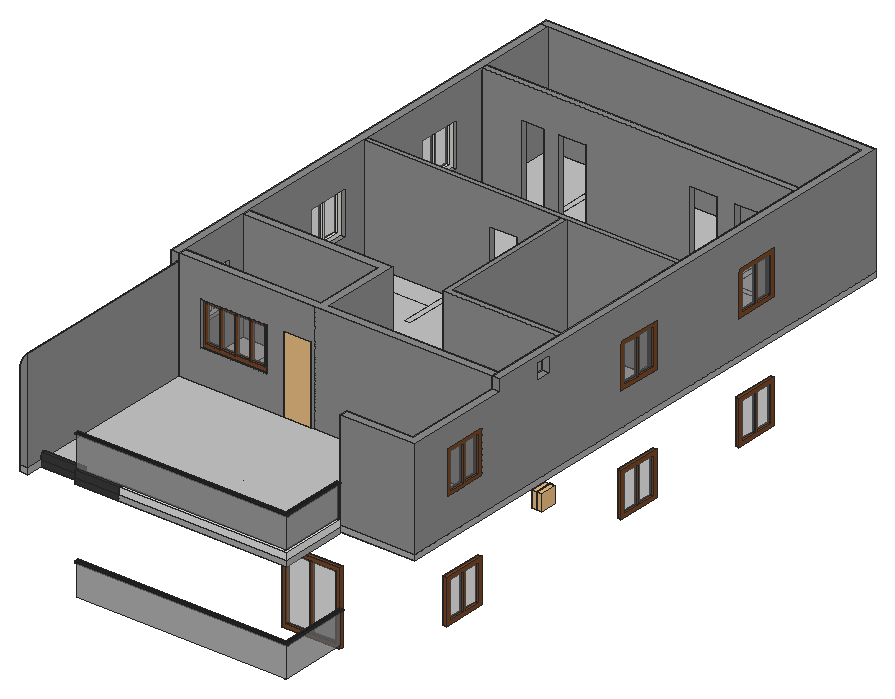
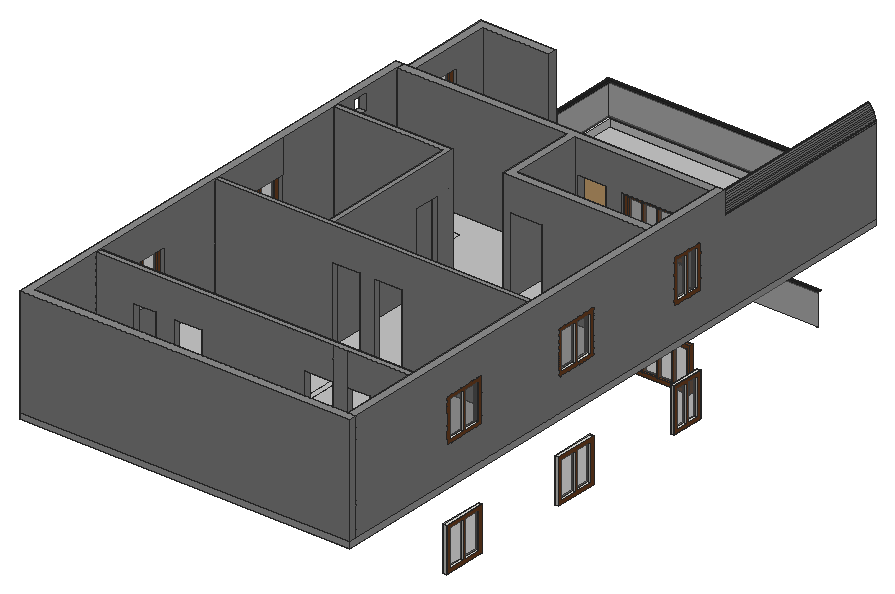
# SketchUp Ruby script. Lengths in inches.
U = 1.inch
M = Sketchup.active_model
def pt(a) = Geom::Point3d.new(a.map { |v| v * U })
def face(e, loops, mat)
  f = e.add_face(loops[0].map { |a| pt(a) })
  loops[1..].each { |l| e.add_face(l.map { |a| pt(a) }).erase! }
  f.material = f.back_material = mat if mat
  f
end
# faces: each face lists its corners as indices into pts; further lists are holes
def faces(e, pts, list, mat = nil) = list.each { |f| face(e, (f[0].is_a?(Array) ? f : [f]).map { |l| l.map { |i| pts[i] } }, mat) }
# xy, xz, yz: faces in a plane at the given z, y or x. An outline is a flat list of corners, or four numbers for a rectangle; further outlines are holes
def ring(l) = l.size == 4 ? [[l[0], l[1]], [l[2], l[1]], [l[2], l[3]], [l[0], l[3]]] : l.each_slice(2).to_a
def flat(e, list, mat, &to3) = list.each { |f| face(e, (f[0].is_a?(Array) ? f : [f]).map { |l| ring(l).map { |u, v| to3.(u, v) } }, mat) }
def xy(e, z, list, mat = nil) = flat(e, list, mat) { |x, y| [x, y, z] }
def xz(e, y, list, mat = nil) = flat(e, list, mat) { |x, z| [x, y, z] }
def yz(e, x, list, mat = nil) = flat(e, list, mat) { |y, z| [x, y, z] }
def lines(e, pts, list) = list.each { |a, b| e.add_line(pt(pts[a]), pt(pts[b])) }
# prism: a flat outline (further loops are holes) pulled along v
def prism(e, loops, v, mat = nil)
  f = face(e, loops, mat); d = Geom::Vector3d.new(v.map { |x| x * U })
  f.pushpull(f.normal.samedirection?(d) ? d.length : -d.length)
end
def box(e, o, s, mat = nil) = prism(e, [[o, [o[0] + s[0], o[1], o[2]], [o[0] + s[0], o[1] + s[1], o[2]], [o[0], o[1] + s[1], o[2]]]], [0, 0, s[2]], mat)
def at(x, y, z, deg = 0) = Geom::Transformation.translation(pt([x, y, z])) * Geom::Transformation.rotation(ORIGIN, Z_AXIS, deg.degrees)
def axes(o, x, y, z) = Geom::Transformation.new([*x, 0, *y, 0, *z, 0, *pt(o).to_a, 1])
def part(name) = M.definitions.add(name)
# library, detail: a bought-in or finely detailed component or shape, given as its bounding box
def library(name, o, s) = part(name).tap { |d| box(d.entities, o, s) }
def detail(e, o, s) = box(e.add_group.entities, o, s)
def put(e, d, t, mat = nil) = e.add_instance(d, t).tap { |i| i.material = mat if mat }
def group(e, t, mat = nil) = e.add_group.tap { |g| g.transformation = t; g.material = mat if mat }.entities
root = M.entities
M.materials.add("[Color M01]").color = [226, 226, 226]
M.materials.add("[Color M02]").color = [198, 198, 198]
M.materials.add("[Color M03]").color = [170, 170, 170]
M.materials.add("[Color M04]").color = [142, 142, 142]
M.materials.add("[Color M07]").color = [58, 58, 58]
M.materials.add("[Color M08]").color = [30, 30, 30]
M.materials.add("[Metal Seamed]").color = [118, 119, 115]
M.materials.add("[Translucent Glass Gray]").color = [128, 128, 128]
M.materials["[Translucent Glass Gray]"].alpha = 0.5
M.materials.add("[Wood Veneer 01]").color = [120, 70, 37]
c1 = part("Group49\#1")
xy(c1.entities,0,[[-27.41,-35.91,-0.59,35.91],[0.59,-35.91,27.41,35.91]])
c2 = part("Group48\#1")
prism(c2.entities,[[[-31.34,39.84,0],[31.34,39.84,0],[31.34,-39.84,0],[-31.34,-39.84,0]],[[27.41,35.91,0],[0.59,35.91,0],[0.59,-35.91,0],[27.41,-35.91,0]],[[-27.41,-35.91,0],[-0.59,-35.91,0],[-0.59,35.91,0],[-27.41,35.91,0]]],[0,0,4],"[Wood Veneer 01]")
put(c2.entities,c1,at(0,0,2),"[Translucent Glass Gray]")
c3 = part("Group19\#1")
xy(c3.entities,0,[[-32.0625,-20.0625,-16.92,20.0625],[-15.73,-20.0625,-0.59,20.0625],[0.59,-20.0625,15.73,20.0625],[16.92,-20.0625,32.0625,20.0625]],"[Translucent Glass Gray]")
c4 = part("Group18\#1")
prism(c4.entities,[[[36,24,0],[36,-24,0],[-36,-24,0],[-36,24,0]],[[-15.73,20.0625,0],[-15.73,-20.0625,0],[-0.59,-20.0625,0],[-0.59,20.0625,0]],[[-32.0625,20.0625,0],[-32.0625,-20.0625,0],[-16.92,-20.0625,0],[-16.92,20.0625,0]],[[0.59,20.0625,0],[0.59,-20.0625,0],[15.73,-20.0625,0],[15.73,20.0625,0]],[[32.0625,20.0625,0],[16.92,20.0625,0],[16.92,-20.0625,0],[32.0625,-20.0625,0]]],[0,0,4],"[Wood Veneer 01]")
put(c4.entities,c3,at(0,0,2))
c5 = part("Group35\#1")
xy(c5.entities,0,[[-20.12,-20.0625,-0.59,20.0625],[0.59,-20.0625,20.12,20.0625]])
c6 = part("Group34\#2")
prism(c6.entities,[[[24.05,24,0],[24.05,-24,0],[-24.05,-24,0],[-24.05,24,0]],[[0.59,-20.0625,0],[20.12,-20.0625,0],[20.12,20.0625,0],[0.59,20.0625,0]],[[-20.12,-20.0625,0],[-0.59,-20.0625,0],[-0.59,20.0625,0],[-20.12,20.0625,0]]],[0,0,4],"[Wood Veneer 01]")
put(c6.entities,c5,at(0,0,2),"[Translucent Glass Gray]")
c7 = part("Group21\#2")
xy(c7.entities,0,[[-20.0625,-20.0625,-0.59,20.0625],[0.59,-20.0625,20.0625,20.0625]])
c8 = part("Group20\#3")
prism(c8.entities,[[[-24,24,0],[24,24,0],[24,-24,0],[-24,-24,0]],[[-20.0625,-20.0625,0],[-0.59,-20.0625,0],[-0.59,20.0625,0],[-20.0625,20.0625,0]],[[20.0625,20.0625,0],[0.59,20.0625,0],[0.59,-20.0625,0],[20.0625,-20.0625,0]]],[0,0,4],"[Wood Veneer 01]")
put(c8.entities,c7,at(0,0,2),"[Translucent Glass Gray]")
c9 = part("Group90\#1")
xy(c9.entities,0,[[-20.0625,-20.0625,-0.59,20.0625],[0.59,-20.0625,20.0625,20.0625]])
c10 = part("Group89\#1")
xy(c10.entities,0,[[[-24,-24,24,24],[-20.0625,-20.0625,-0.59,20.0625],[0.59,-20.0625,20.0625,20.0625]]])
xy(c10.entities,4,[[[-24,-24,24,24],[-20.0625,-20.0625,-0.59,20.0625],[0.59,-20.0625,20.0625,20.0625]]],"[Wood Veneer 01]")
xz(c10.entities,-24,[[-24,0,24,4]])
xz(c10.entities,-20.0625,[[-20.0625,0,-0.59,4],[0.59,0,20.0625,4]])
xz(c10.entities,20.0625,[[-20.0625,0,-0.59,4],[0.59,0,20.0625,4]])
xz(c10.entities,24,[[-24,0,24,4]])
yz(c10.entities,-24,[[-24,0,24,4]])
yz(c10.entities,-20.0625,[[-20.0625,0,20.0625,4]])
yz(c10.entities,-0.59,[[-20.0625,0,20.0625,4]])
yz(c10.entities,0.59,[[-20.0625,0,20.0625,4]])
yz(c10.entities,20.0625,[[-20.0625,0,20.0625,4]])
yz(c10.entities,24,[[-24,0,24,4]])
put(c10.entities,c9,at(0,0,2),"[Translucent Glass Gray]")
c11 = part("Group92\#1")
xy(c11.entities,0,[[-14.01,-20.0625,-0.59,20.0625],[0.59,-20.0625,14.01,20.0625]])
c12 = part("Group91\#1")
xy(c12.entities,0,[[[-17.94,-24,17.94,24],[0.59,-20.0625,14.01,20.0625],[-14.01,-20.0625,-0.59,20.0625]]])
xy(c12.entities,4,[[[-17.94,-24,17.94,24],[0.59,-20.0625,14.01,20.0625],[-14.01,-20.0625,-0.59,20.0625]]],"[Wood Veneer 01]")
xz(c12.entities,-24,[[-17.94,0,17.94,4]])
xz(c12.entities,-20.0625,[[-14.01,0,-0.59,4],[0.59,0,14.01,4]])
xz(c12.entities,20.0625,[[-14.01,0,-0.59,4],[0.59,0,14.01,4]])
xz(c12.entities,24,[[-17.94,0,17.94,4]])
yz(c12.entities,-17.94,[[-24,0,24,4]])
yz(c12.entities,-14.01,[[-20.0625,0,20.0625,4]])
yz(c12.entities,-0.59,[[-20.0625,0,20.0625,4]])
yz(c12.entities,0.59,[[-20.0625,0,20.0625,4]])
yz(c12.entities,14.01,[[-20.0625,0,20.0625,4]])
yz(c12.entities,17.94,[[-24,0,24,4]])
put(c12.entities,c11,at(0,0,2),"[Translucent Glass Gray]")
c13 = library("Agrupar\#12",[-0.01,0,0],[12.55,78.74,39.39])
c14 = part("Union\#1")
xy(c14.entities,0,[[[0,0,0,719,360.05,719,360.05,89,278.76,89,278.76,85.74,153.74,85.74,153.74,202.74,102.11,202.74,102.11,19.26,278.76,19.26,278.76,85,282.03,85,282.03,12,51,12,51,18,9,18,9,0],[13,20,94.84,202]]])
xy(c14.entities,3,[[102.11,19.26,102.11,202.74,153.74,202.74,153.74,85.74,278.76,85.74,278.76,19.26],[13,20,94.84,202]],"[Color M07]")
xy(c14.entities,6,[[0,0,9,0,9,18,51,18,51,12,98.84,12,98.84,16,278.03,16,278.03,85,278.76,85,278.76,89,360.05,89,360.05,719,0,719]],"[Color M02]")
xy(c14.entities,14,[[98.84,12,282.03,12,282.03,85,278.03,85,278.03,16,98.84,16]],"[Color M01]")
xz(c14.entities,0,[[0,0,9,6]])
xz(c14.entities,12,[[98.84,0,282.03,6]])
xz(c14.entities,12,[[98.84,6,282.03,14]],"[Color M01]")
xz(c14.entities,12,[[51,0,98.84,6]],"[Color M07]")
xz(c14.entities,16,[[98.84,6,278.03,14]],"[Color M01]")
xz(c14.entities,18,[[9,0,51,6]],"[Color M07]")
xz(c14.entities,19.26,[[102.11,0,278.76,3]],"[Color M07]")
xz(c14.entities,20,[[13,0,94.84,3]],"[Color M07]")
xz(c14.entities,85,[[278.76,0,282.03,6]])
xz(c14.entities,85,[[278.03,6,282.03,14]],"[Color M01]")
xz(c14.entities,85.74,[[153.74,0,278.76,3]],"[Color M07]")
xz(c14.entities,89,[[278.76,0,360.05,6]])
xz(c14.entities,202,[[13,0,94.84,3]],"[Color M07]")
xz(c14.entities,202.74,[[102.11,0,153.74,3]],"[Color M07]")
xz(c14.entities,719,[[0,0,360.05,6]])
yz(c14.entities,0,[[0,0,719,6]])
yz(c14.entities,9,[[0,0,18,6]])
yz(c14.entities,13,[[20,0,202,3]],"[Color M07]")
yz(c14.entities,51,[[12,0,18,6]],"[Color M07]")
yz(c14.entities,94.84,[[20,0,202,3]],"[Color M07]")
yz(c14.entities,98.84,[[12,6,16,14]],"[Color M01]")
yz(c14.entities,102.11,[[19.26,0,202.74,3]],"[Color M07]")
yz(c14.entities,153.74,[[85.74,0,202.74,3]],"[Color M07]")
yz(c14.entities,278.03,[[16,6,85,14]],"[Color M01]")
yz(c14.entities,278.76,[[85.74,0,89,0,89,6,85,6,85,3,85.74,3]])
yz(c14.entities,278.76,[[19.26,0,85,3],[85,0,85.74,3]],"[Color M07]")
yz(c14.entities,282.03,[[12,0,85,6]])
yz(c14.entities,282.03,[[12,6,85,14]],"[Color M01]")
yz(c14.entities,360.05,[[89,0,719,6]])
c15 = library("PINTU 6 YA",[0,-0.6875,0],[35.83,8.07,80.71])
p = [[278.03,133.1875,210],[215.34,133.1875,210],[215.34,133.1875,130.3125],[278.03,133.1875,130.3125],[0,629.94,162],[0,629.94,210],
  [0,581.94,210],[0,581.94,162],[0,283.65,210],[0,319.54,210],[0,319.54,162],[0,283.65,162],
  [98.84,60.1875,260],[98.84,60.1875,246]]
lines(root,p,[[0,1],[1,2],[2,3],[3,0],[4,5],[5,6],[6,7],[7,4],[8,9],[9,10],[10,11],[11,8],
  [12,13]])
put(root,c2,axes([246.68,137.1875,170.16],[1,0,0],[0,0,1],[0,-1,0]))
g1 = group(root,at(51,56.1875,134.1875),"[Color M07]")
g2 = group(g1,at(0,0,35.1875),"[Color M08]")
xy(g2,-0.02,[[231.14,0,231.19,77],[231.19,0,231.25,77]])
xy(g2,0,[[0,0,0,4,227.03,4,227.03,77,231.03,77,231.03,0]])
xy(g2,1.5,[[0,0,231.03,0,231.03,77,227.03,77,227.03,4,0,4]])
xy(g2,1.52,[[231.14,0,231.19,77],[231.19,0,231.25,77]])
xz(g2,0,[[231.14,-0.02,231.25,-0.02,231.35,0,231.41,0.01,231.51,0.05,231.5625,0.07,231.61,0.1,231.65,0.13,231.7,0.17,231.74,0.2,231.78,0.24,231.81,0.29,231.84,0.33,231.87,0.38,231.89,0.43,231.92,0.48,231.93,0.53,231.95,0.59,231.96,0.64,231.96,0.86,231.95,0.91,231.93,0.97,231.92,1.02,231.89,1.07,231.87,1.12,231.84,1.17,231.81,1.21,231.78,1.26,231.74,1.3,231.7,1.33,231.65,1.37,231.61,1.4,231.5625,1.43,231.51,1.45,231.41,1.49,231.35,1.5,231.25,1.52,231.14,1.52,231.08,1.51,231.03,1.5,231.03,0,231.08,-0.01],[0,0,231.03,1.5]])
xz(g2,4,[[0,0,227.03,1.5]])
xz(g2,77,[[231.14,-0.02,231.08,-0.01,231.03,0,231.03,1.5,231.08,1.51,231.14,1.52,231.25,1.52,231.35,1.5,231.41,1.49,231.51,1.45,231.5625,1.43,231.61,1.4,231.65,1.37,231.7,1.33,231.74,1.3,231.78,1.26,231.81,1.21,231.84,1.17,231.87,1.12,231.89,1.07,231.92,1.02,231.93,0.97,231.95,0.91,231.96,0.86,231.96,0.64,231.95,0.59,231.93,0.53,231.92,0.48,231.89,0.43,231.87,0.38,231.84,0.33,231.81,0.29,231.78,0.24,231.74,0.2,231.7,0.17,231.65,0.13,231.61,0.1,231.5625,0.07,231.51,0.05,231.41,0.01,231.35,0,231.25,-0.02],[227.03,0,231.03,1.5]])
yz(g2,0,[[0,0,4,1.5]])
yz(g2,227.03,[[4,0,77,1.5]])
yz(g2,231.96,[[0,0.64,77,0.69],[0,0.69,77,0.75],[0,0.75,77,0.81],[0,0.81,77,0.86]])
p = [[231.08,0,-0.01],[231.03,0,0],[231.03,77,0],[231.08,77,-0.01],[231.14,0,-0.02],[231.14,77,-0.02],
  [231.3,0,-0.01],[231.25,0,-0.02],[231.25,77,-0.02],[231.3,77,-0.01],[231.35,0,0],[231.35,77,0],
  [231.46,0,0.03],[231.41,0,0.01],[231.41,77,0.01],[231.46,77,0.03],[231.5625,0,0.07],[231.51,0,0.05],
  [231.51,77,0.05],[231.5625,77,0.07],[231.65,0,0.13],[231.61,0,0.1],[231.61,77,0.1],[231.65,77,0.13],
  [231.7,0,0.17],[231.7,77,0.17],[231.78,0,0.24],[231.74,0,0.2],[231.74,77,0.2],[231.78,77,0.24],
  [231.81,0,0.29],[231.81,77,0.29],[231.87,0,0.38],[231.84,0,0.33],[231.84,77,0.33],[231.87,77,0.38],
  [231.92,0,0.48],[231.89,0,0.43],[231.89,77,0.43],[231.92,77,0.48],[231.95,0,0.59],[231.93,0,0.53],
  [231.93,77,0.53],[231.95,77,0.59],[231.96,0,0.64],[231.96,77,0.64],[231.95,0,0.91],[231.96,0,0.86],
  [231.96,77,0.86],[231.95,77,0.91],[231.93,0,0.97],[231.93,77,0.97],[231.92,0,1.02],[231.92,77,1.02],
  [231.89,0,1.07],[231.89,77,1.07],[231.84,0,1.17],[231.87,0,1.12],[231.87,77,1.12],[231.84,77,1.17],
  [231.78,0,1.26],[231.81,0,1.21],[231.81,77,1.21],[231.78,77,1.26],[231.7,0,1.33],[231.74,0,1.3],
  [231.74,77,1.3],[231.7,77,1.33],[231.65,0,1.37],[231.65,77,1.37],[231.51,0,1.45],[231.5625,0,1.43],
  [231.5625,77,1.43],[231.51,77,1.45],[231.61,0,1.4],[231.61,77,1.4],[231.03,0,1.5],[231.08,0,1.51],
  [231.08,77,1.51],[231.03,77,1.5],[231.14,0,1.52],[231.14,77,1.52],[231.25,0,1.52],[231.3,0,1.51],
  [231.3,77,1.51],[231.25,77,1.52],[231.35,0,1.5],[231.35,77,1.5],[231.41,0,1.49],[231.46,0,1.47],
  [231.46,77,1.47],[231.41,77,1.49]]
faces(g2,p,[[0,1,2,3],[4,0,3,5],[6,7,8,9],[10,6,9,11],[12,13,14,15],[13,10,11,14],[16,17,18,19],[17,12,15,18],
  [20,21,22,23],[21,16,19,22],[24,20,23,25],[26,27,28,29],[27,24,25,28],[30,26,29,31],[32,33,34,35],[33,30,31,34],
  [36,37,38,39],[37,32,35,38],[40,41,42,43],[41,36,39,42],[44,40,43,45],[46,47,48,49],[50,46,49,51],[52,50,51,53],
  [54,52,53,55],[56,57,58,59],[57,54,55,58],[60,61,62,63],[61,56,59,62],[64,65,66,67],[65,60,63,66],[68,64,67,69],
  [70,71,72,73],[74,68,69,75],[71,74,75,72],[76,77,78,79],[77,80,81,78],[82,83,84,85],[83,86,87,84],[88,89,90,91],
  [86,88,91,87],[89,70,73,90]])
g3 = group(g1,at(0,2,0.6875),"[Metal Seamed]")
prism(g3,[[[0,0,-0.6875],[0,0.26,-0.6875],[228.77,0.26,-0.6875],[228.77,75,-0.6875],[229.03,75,-0.6875],[229.03,0,-0.6875]]],[0,0,35.1875],"[Translucent Glass Gray]")
put(root,c4,axes([69,256.5,186],[1,0,0],[0,0,1],[0,-1,0]))
put(root,c6,axes([161,214.38,186],[0,-1,0],[0,0,1],[-1,0,0]))
put(root,c8,axes([356.05,201.2,186],[0,1,0],[0,0,1],[1,0,0]))
put(root,c10,axes([4,605.94,186],[0,-1,0],[0,0,1],[-1,0,0]))
put(root,c10,axes([4,453.75,186],[0,-1,0],[0,0,1],[-1,0,0]))
put(root,c12,axes([4,301.6,186],[0,-1,0],[0,0,1],[-1,0,0]))
put(root,c8,axes([356.05,439.46,186],[0,1,0],[0,0,1],[1,0,0]))
put(root,c8,axes([356.05,600.375,186],[0,1,0],[0,0,1],[1,0,0]))
put(root,c13,axes([354.41,318.42,222],[0.45,0,0],[0,-0.2286,0],[0,0,0.45697]))
put(root,c13,axes([365.07,318.42,222],[-0.45,0,0],[0,-0.2286,0],[0,0,0.45697]))
g4 = group(root,at(0,44.1875,246),"[Color M03]")
p = [[98.84,16,14],[98.84,16,0],[98.26,16,14]]
lines(g4,p,[[0,1],[2,0]])
put(g4,c14,at(0,0,0))
g5 = group(g4,at(98.84,16,6))
prism(g5,[[[-47.84,-4,0],[-47.84,2,0],[-89.84,2,0],[-89.84,6,0],[-43.84,6,0],[-43.84,0,0],[0,0,0],[0,-4,0]]],[0,0,8],"[Color M07]")
g6 = group(root,at(0,44.1875,252),"[Color M04]")
xy(g6,0,[[0,0,9,239.47],[278.78,89,351.05,98],[351.05,89,360.05,371.28],[9,206,123.49,215],[153.49,206,157,215],
  [157,206,157,302,166,302,166,215,351.05,215,351.05,206],[0,239.47,9,385.56],[9,293,123.07,302],[225.05,296,351.05,302],[225.05,302,231.05,317.31],
  [225.05,347.31,231.05,458],[9,458,146.57,464],[176.57,458,192.16,464],[222.16,458,351.05,464],[351.05,532.1875,351.05,710,273,710,273,719,360.05,719,360.05,532.1875],
  [0,537.75,0,719,87,719,87,710,9,710,9,537.75],[9,620,52.02,626],[76.02,620,92.56,626],[122.56,620,235.54,626],[265.54,620,285.72,626],
  [309.72,620,351.05,626]])
xy(g6,36,[[351.05,133.01,360.05,181.01],[33,206,105,215],[0,239.47,9,275.35],[351.05,371.28,360.05,419.28],[0,385.56,9,433.56],
  [351.05,532.1875,360.05,580.1875],[0,537.75,9,585.75]])
xy(g6,84,[[351.05,133.01,360.05,181.01],[33,206,105,215],[123.49,206,153.49,215],[0,239.47,9,275.35],[123.07,293,157,302],
  [225.05,317.31,231.05,347.31],[351.05,371.28,360.05,419.28],[0,385.56,9,433.56],[146.57,458,176.57,464],[192.16,458,222.16,464],
  [351.05,532.1875,360.05,580.1875],[0,537.75,9,585.75],[52.02,620,76.02,626],[92.56,620,122.56,626],[235.54,620,265.54,626],
  [285.72,620,309.72,626]])
xy(g6,96,[[351.05,256.23,360.05,274.23]])
xy(g6,107.9375,[[278.78,89,360.05,89,360.05,206,351.05,206,351.05,98,278.78,98]])
xy(g6,114,[[351.05,256.23,360.05,274.23]])
xy(g6,120,[[0,206,9,710],[351.05,206,360.05,206,360.05,719,0,719,0,710,351.05,710],[9,206,351.05,206,351.05,215,166,215,166,302,9,302,9,293,157,293,157,215,9,215],[225.05,296,351.05,296,351.05,302,231.05,302,231.05,458,225.05,458],[9,458,351.05,464],
  [9,620,351.05,626]])
xz(g6,0,[[0,0,9,0,9,112.72,8.15,111.92,8.11,111.89,8.1,111.87,6.91,110.61,5.79,109.25,4.76,107.83,3.82,106.35,2.98,104.8125,2.23,103.23,1.58,101.59,1.04,99.93,0.6,98.23,0.28,96.5,0.11,95.17,0,94.05],[0.06,94.76,0.11,95.17,0.15,95.63],[0.11,95.17,0.28,96.5,0.6,98.23,1.04,99.93,1.58,101.59,2.23,103.23,2.98,104.8125,3.82,106.35,4.76,107.83,5.79,109.25,6.91,110.61,8.1,111.87,7.54,111.32,6.4,110.08,5.35,108.76,4.38,107.38,3.5,105.94,2.71,104.45,2.02,102.92,1.42,101.34,0.93,99.73,0.53,98.09,0.24,96.43,0.15,95.63]])
xz(g6,89,[[278.78,0,360.05,107.9375]])
xz(g6,98,[[278.78,0,351.05,107.9375]])
xz(g6,133.01,[[351.05,36,360.05,84]])
xz(g6,181.01,[[351.05,36,360.05,84]])
xz(g6,206,[[[9,0,123.49,0,123.49,84,153.49,84,153.49,0,157,0,157,120,9,120],[33,36,105,84]],[157,0,351.05,120],[0,94.05,0.11,95.17,0.06,94.76,0.15,95.63,0.24,96.43,0.53,98.09,0.93,99.73,1.42,101.34,2.02,102.92,2.71,104.45,3.5,105.94,4.38,107.38,5.35,108.76,6.4,110.08,7.54,111.32,8.1,111.87,8.11,111.89,8.15,111.92,9,112.72,9,120,0,120],[351.05,107.9375,360.05,120]])
xz(g6,215,[[[9,0,9,120,157,120,157,0,153.49,0,153.49,84,123.49,84,123.49,0],[33,36,105,84]],[166,0,351.05,120]])
xz(g6,239.47,[[0,36,9,84]])
xz(g6,256.23,[[351.05,96,360.05,114]])
xz(g6,274.23,[[351.05,96,360.05,114]])
xz(g6,275.35,[[0,36,9,84]])
xz(g6,293,[[9,0,123.07,0,123.07,84,157,84,157,120,9,120]])
xz(g6,296,[[225.05,0,351.05,120]])
xz(g6,302,[[9,0,9,120,166,120,166,0,157,0,157,84,123.07,84,123.07,0],[231.05,0,351.05,120]])
xz(g6,317.31,[[225.05,0,231.05,84]])
xz(g6,347.31,[[225.05,0,231.05,84]])
xz(g6,371.28,[[351.05,36,360.05,84]])
xz(g6,385.56,[[0,36,9,84]])
xz(g6,419.28,[[351.05,36,360.05,84]])
xz(g6,433.56,[[0,36,9,84]])
xz(g6,458,[[9,0,146.57,0,146.57,84,176.57,84,176.57,0,192.16,0,192.16,84,222.16,84,222.16,0,225.05,0,225.05,120,9,120],[225.05,0,231.05,120],[231.05,0,351.05,120]])
xz(g6,464,[[9,0,9,120,351.05,120,351.05,0,222.16,0,222.16,84,192.16,84,192.16,0,176.57,0,176.57,84,146.57,84,146.57,0]])
xz(g6,532.1875,[[351.05,36,360.05,84]])
xz(g6,537.75,[[0,36,9,84]])
xz(g6,580.1875,[[351.05,36,360.05,84]])
xz(g6,585.75,[[0,36,9,84]])
xz(g6,620,[[9,0,52.02,0,52.02,84,76.02,84,76.02,0,92.56,0,92.56,84,122.56,84,122.56,0,235.54,0,235.54,84,265.54,84,265.54,0,285.72,0,285.72,84,309.72,84,309.72,0,351.05,0,351.05,120,9,120]])
xz(g6,626,[[9,0,9,120,76.02,120,76.02,84,52.02,84,52.02,0],[76.02,0,92.56,120],[122.56,0,122.56,84,92.56,84,92.56,120,351.05,120,351.05,0,309.72,0,309.72,84,285.72,84,285.72,0,265.54,0,265.54,84,235.54,84,235.54,0]])
xz(g6,710,[[9,0,351.05,120]])
xz(g6,719,[[0,0,360.05,120]])
yz(g6,0,[[[0,0,0,94.05,206,94.05,206,120,710,120,710,0],[537.75,36,585.75,84],[385.56,36,433.56,84],[239.47,36,275.35,84]],[710,0,719,120]])
yz(g6,9,[[0,0,206,112.72],[206,0,215,120],[[215,0,293,120],[239.47,36,275.35,84]],[293,0,302,120],[[302,0,458,120],[385.56,36,433.56,84]],
  [458,0,464,120],[[464,0,620,120],[537.75,36,585.75,84]],[620,0,626,120],[626,0,710,120]])
yz(g6,33,[[206,36,215,84]])
yz(g6,52.02,[[620,0,626,84]])
yz(g6,76.02,[[620,0,626,84]])
yz(g6,92.56,[[620,0,626,84]])
yz(g6,105,[[206,36,215,84]])
yz(g6,122.56,[[620,0,626,84]])
yz(g6,123.07,[[293,0,302,84]])
yz(g6,123.49,[[206,0,215,84]])
yz(g6,146.57,[[458,0,464,84]])
yz(g6,153.49,[[206,0,215,84]])
yz(g6,157,[[215,0,215,120,293,120,293,84,302,84,302,0]])
yz(g6,166,[[215,0,302,120]])
yz(g6,176.57,[[458,0,464,84]])
yz(g6,192.16,[[458,0,464,84]])
yz(g6,222.16,[[458,0,464,84]])
yz(g6,225.05,[[296,0,296,120,458,120,458,0,347.31,0,347.31,84,317.31,84,317.31,0]])
yz(g6,231.05,[[302,0,317.31,0,317.31,84,347.31,84,347.31,0,458,0,458,120,302,120]])
yz(g6,235.54,[[620,0,626,84]])
yz(g6,265.54,[[620,0,626,84]])
yz(g6,278.78,[[89,0,98,107.9375]])
yz(g6,285.72,[[620,0,626,84]])
yz(g6,309.72,[[620,0,626,84]])
yz(g6,351.05,[[[98,0,206,107.9375],[133.01,36,181.01,84]],[206,0,215,120],[[215,0,296,120],[256.23,96,274.23,114]],[296,0,302,120],[302,0,371.28,120],
  [371.28,0,371.28,36,419.28,36,419.28,84,371.28,84,371.28,120,458,120,458,0],[458,0,464,120],[[464,0,620,120],[532.1875,36,580.1875,84]],[620,0,626,120],[626,0,710,120]])
yz(g6,360.05,[[[89,0,719,0,719,120,206,120,206,107.9375,89,107.9375],[532.1875,36,580.1875,84],[133.01,36,181.01,84],[371.28,36,419.28,84],[256.23,96,274.23,114]]])
p = [[0,0,94.05],[0.11,0,95.17],[0.11,206,95.17],[0,206,94.05],[0.06,0,94.76],[0.06,206,94.76],
  [0.15,0,95.63],[0.15,206,95.63],[0.24,0,96.43],[0.24,206,96.43],[0.53,0,98.09],[0.53,206,98.09],
  [0.93,0,99.73],[0.93,206,99.73],[1.42,0,101.34],[1.42,206,101.34],[2.02,0,102.92],[2.02,206,102.92],
  [2.71,0,104.45],[2.71,206,104.45],[3.5,0,105.94],[3.5,206,105.94],[4.38,0,107.38],[4.38,206,107.38],
  [5.35,0,108.76],[5.35,206,108.76],[6.4,0,110.08],[6.4,206,110.08],[7.54,0,111.32],[7.54,206,111.32],
  [8.1,0,111.87],[8.1,206,111.87],[8.11,0,111.89],[8.11,206,111.89],[8.15,0,111.92],[8.15,206,111.92],
  [9,0,112.72],[9,206,112.72],[45,257,0],[45,293,0],[222.13,464,0],[222.16,464,0],
  [261.05,296,0],[261.05,242,0],[153.07,302,0],[157,302,0],[182,620,0],[182,464,0],
  [105.05,353.74,0],[105.05,302,0],[188,620,0],[188,464,0],[81,710,0],[81,626,0],
  [273,710,0],[273,626,0],[9,257,0],[9,251,0],[45,251,0],[87,710,0],
  [87,626,0],[267.05,296,0],[267.05,248,0],[279,710,0],[279,626,0],[166,98,0],
  [166.0625,98,0],[75,257,0],[75,293,0],[99,458,0],[99,434,0],[99,353.74,0],
  [99,302,0],[105.05,458,0],[105.05,401.74,0],[122.52,626,0],[122.56,626,0],[105,251,0],
  [105,232.1875,0],[65,257,0],[65,293,0],[85,257,0],[85,293,0],[65,251,0],
  [65,232.1875,0],[37.2,234.69,0],[37.2,232.1875,0],[37.2,229.73,0],[33.94,232.1875,0],[55,257,0],
  [55,293,0],[85,251,0],[85,232.1875,0],[71.09,229.73,0],[67.84,232.1875,0],[95,257,0],
  [95,293,0],[71.09,234.69,0],[71.09,232.1875,0],[95,251,0],[95,232.1875,0],[115,251,0],
  [115,257,0],[75,251,0],[75,232.1875,0],[117.74,232.1875,0],[55,251,0],[55,232.1875,0],
  [231.05,302,84],[225.05,302,84],[153.07,293,0],[157,293,0],[222.16,458,0],[105,257,0],
  [105,293,0],[45,232.1875,0],[44.11,434,0],[44.11,302,0],[99,401.74,0],[75,215,0],
  [122.52,620,0],[123.49,215,0],[123.83,215,0],[65,215,0],[95,215,0],[231.05,347.31,0],
  [231.05,347.27,0],[105,215,0],[146.57,464,0],[146.61,464,0],[52.02,620,0],[76.02,620,0],
  [123.49,206,0],[153.49,206,0],[45,215,0],[122.56,620,0],[34.15,232.1875,0],[235.54,626,0],
  [235.58,626,0],[115,293,0],[225.05,347.31,0],[225.05,317.31,0],[123.07,302,0],[123.41,302,0],
  [85,215,0],[55,215,0],[192.16,458,0],[123.07,293,0],[146.57,458,0],[176.57,458,0],
  [235.54,620,0],[265.54,620,0],[285.72,626,0],[309.72,626,0],[92.56,620,0],[285.72,620,0],
  [309.72,620,0],[351.05,242,0],[351.05,248,0],[9.39,0,113.09],[8.74,0,112.5]]
faces(g6,p,[[0,1,2,3],[1,4,5,2],[4,6,7,5],[6,8,9,7],[8,10,11,9],[10,12,13,11],[12,14,15,13],[14,16,17,15],
  [16,18,19,17],[18,20,21,19],[20,22,23,21],[22,24,25,23],[24,26,27,25],[26,28,29,27],[28,30,31,29],[30,32,33,31],
  [32,34,35,33],[34,36,37,35]])
lines(g6,p,[[38,39],[40,41],[42,43],[44,45],[46,47],[48,49],[50,51],[52,53],[54,55],[56,38],[57,58],[59,60],
  [61,62],[63,64],[65,66],[67,68],[69,70],[71,72],[73,74],[75,76],[77,78],[79,80],[81,82],[83,84],
  [85,86],[87,88],[89,90],[91,92],[93,94],[95,96],[88,85],[97,98],[99,100],[101,102],[103,104],[105,78],
  [106,107],[108,109],[48,71],[110,111],[112,40],[113,114],[58,115],[94,97],[116,117],[118,74],[70,116],[67,81],
  [99,77],[38,89],[92,104],[78,100],[104,119],[75,120],[121,122],[84,123],[100,124],[98,94],[110,44],[125,126],
  [78,127],[58,106],[128,129],[98,93],[86,87],[130,131],[132,133],[115,134],[120,135],[103,91],[94,84],[86,136],
  [137,138],[102,139],[84,107],[115,86],[107,115],[100,92],[140,141],[81,95],[79,67],[142,143],[92,144],[107,145],
  [70,118],[104,98],[146,112],[89,79],[83,103],[147,110],[77,101],[148,149],[150,151],[95,113],[91,99],[113,102],
  [106,83],[152,153],[154,120],[155,156],[43,157],[62,158],[159,36],[160,34]])
put(root,c15,axes([123.49,250.25,252],[0.83729,0,0],[0,0.08537,0],[0,0,1.04078]))
g7 = group(root,at(51,56.1875,260),"[Color M07]")
g8 = group(g7,at(0,0,35.1875),"[Color M08]")
xy(g8,-0.02,[[231.14,0,231.19,72.98],[231.19,0,231.25,72.98]])
xy(g8,0,[[0,0,0,4,227.03,4,227.03,72.98,231.03,72.98,231.03,0]])
xy(g8,1.5,[[0,0,231.03,0,231.03,72.98,227.03,72.98,227.03,4,0,4]])
xy(g8,1.52,[[231.14,0,231.19,72.98],[231.19,0,231.25,72.98]])
xz(g8,0,[[231.14,-0.02,231.25,-0.02,231.35,0,231.41,0.01,231.51,0.05,231.5625,0.07,231.61,0.1,231.65,0.13,231.7,0.17,231.74,0.2,231.78,0.24,231.81,0.29,231.84,0.33,231.87,0.38,231.89,0.43,231.92,0.48,231.93,0.53,231.95,0.59,231.96,0.64,231.96,0.86,231.95,0.91,231.93,0.97,231.92,1.02,231.89,1.07,231.87,1.12,231.84,1.17,231.81,1.21,231.78,1.26,231.74,1.3,231.7,1.33,231.65,1.37,231.61,1.4,231.5625,1.43,231.51,1.45,231.41,1.49,231.35,1.5,231.25,1.52,231.14,1.52,231.08,1.51,231.03,1.5,231.03,0,231.08,-0.01],[0,0,231.03,1.5]])
xz(g8,4,[[0,0,227.03,1.5]])
xz(g8,72.98,[[231.14,-0.02,231.08,-0.01,231.03,0,231.03,1.5,231.08,1.51,231.14,1.52,231.25,1.52,231.35,1.5,231.41,1.49,231.51,1.45,231.5625,1.43,231.61,1.4,231.65,1.37,231.7,1.33,231.74,1.3,231.78,1.26,231.81,1.21,231.84,1.17,231.87,1.12,231.89,1.07,231.92,1.02,231.93,0.97,231.95,0.91,231.96,0.86,231.96,0.64,231.95,0.59,231.93,0.53,231.92,0.48,231.89,0.43,231.87,0.38,231.84,0.33,231.81,0.29,231.78,0.24,231.74,0.2,231.7,0.17,231.65,0.13,231.61,0.1,231.5625,0.07,231.51,0.05,231.41,0.01,231.35,0,231.25,-0.02],[227.03,0,231.03,1.5]])
yz(g8,0,[[0,0,4,1.5]])
yz(g8,227.03,[[4,0,72.98,1.5]])
yz(g8,231.96,[[0,0.64,72.98,0.69],[0,0.69,72.98,0.75],[0,0.75,72.98,0.81],[0,0.81,72.98,0.86]])
p = [[231.03,72.98,0],[231.08,72.98,-0.01],[231.08,0,-0.01],[231.03,0,0],[231.14,72.98,-0.02],[231.14,0,-0.02],
  [231.25,72.98,-0.02],[231.3,72.98,-0.01],[231.3,0,-0.01],[231.25,0,-0.02],[231.35,72.98,0],[231.35,0,0],
  [231.41,72.98,0.01],[231.46,72.98,0.03],[231.46,0,0.03],[231.41,0,0.01],[231.51,72.98,0.05],[231.5625,72.98,0.07],
  [231.5625,0,0.07],[231.51,0,0.05],[231.61,72.98,0.1],[231.65,72.98,0.13],[231.65,0,0.13],[231.61,0,0.1],
  [231.7,72.98,0.17],[231.7,0,0.17],[231.74,0,0.2],[231.74,72.98,0.2],[231.78,72.98,0.24],[231.78,0,0.24],
  [231.81,72.98,0.29],[231.81,0,0.29],[231.84,0,0.33],[231.84,72.98,0.33],[231.87,72.98,0.38],[231.87,0,0.38],
  [231.89,72.98,0.43],[231.89,0,0.43],[231.92,72.98,0.48],[231.92,0,0.48],[231.93,72.98,0.53],[231.93,0,0.53],
  [231.95,72.98,0.59],[231.95,0,0.59],[231.96,72.98,0.64],[231.96,0,0.64],[231.96,0,0.86],[231.96,72.98,0.86],
  [231.95,72.98,0.91],[231.95,0,0.91],[231.93,72.98,0.97],[231.93,0,0.97],[231.92,72.98,1.02],[231.92,0,1.02],
  [231.89,72.98,1.07],[231.89,0,1.07],[231.87,0,1.12],[231.87,72.98,1.12],[231.84,72.98,1.17],[231.84,0,1.17],
  [231.81,0,1.21],[231.81,72.98,1.21],[231.78,72.98,1.26],[231.78,0,1.26],[231.7,0,1.33],[231.74,0,1.3],
  [231.74,72.98,1.3],[231.7,72.98,1.33],[231.65,0,1.37],[231.65,72.98,1.37],[231.51,0,1.45],[231.5625,0,1.43],
  [231.5625,72.98,1.43],[231.51,72.98,1.45],[231.61,0,1.4],[231.61,72.98,1.4],[231.03,0,1.5],[231.08,0,1.51],
  [231.08,72.98,1.51],[231.03,72.98,1.5],[231.14,0,1.52],[231.14,72.98,1.52],[231.25,0,1.52],[231.3,0,1.51],
  [231.3,72.98,1.51],[231.25,72.98,1.52],[231.35,0,1.5],[231.35,72.98,1.5],[231.41,0,1.49],[231.46,0,1.47],
  [231.46,72.98,1.47],[231.41,72.98,1.49]]
faces(g8,p,[[0,1,2,3],[1,4,5,2],[6,7,8,9],[7,10,11,8],[12,13,14,15],[10,12,15,11],[16,17,18,19],[13,16,19,14],
  [20,21,22,23],[17,20,23,18],[21,24,25,22],[26,27,28,29],[24,27,26,25],[29,28,30,31],[32,33,34,35],[31,30,33,32],
  [35,34,36,37],[37,36,38,39],[39,38,40,41],[41,40,42,43],[43,42,44,45],[46,47,48,49],[49,48,50,51],[51,50,52,53],
  [53,52,54,55],[56,57,58,59],[55,54,57,56],[60,61,62,63],[59,58,61,60],[64,65,66,67],[63,62,66,65],[68,64,67,69],
  [70,71,72,73],[74,68,69,75],[71,74,75,72],[76,77,78,79],[77,80,81,78],[82,83,84,85],[83,86,87,84],[88,89,90,91],
  [86,88,91,87],[89,70,73,90]])
g9 = group(g7,at(0,2,0.6875),"[Metal Seamed]")
prism(g9,[[[0,0.26,-0.6875],[228.77,0.26,-0.6875],[228.77,71.1875,-0.6875],[229.03,71.1875,-0.6875],[229.03,0,-0.6875],[0,0,-0.6875]]],[0,0,35.1875],"[Translucent Glass Gray]")
put(root,c8,axes([356.05,439.46,312],[0,1,0],[0,0,1],[1,0,0]))
put(root,c8,axes([356.05,600.375,312],[0,1,0],[0,0,1],[1,0,0]))
put(root,c10,axes([4,453.75,312],[0,-1,0],[0,0,1],[-1,0,0]))
put(root,c10,axes([4,605.94,312],[0,-1,0],[0,0,1],[-1,0,0]))
put(root,c12,axes([4,301.6,312],[0,-1,0],[0,0,1],[-1,0,0]))
put(root,c4,axes([69,256.5,312],[1,0,0],[0,0,1],[0,-1,0]))
put(root,c8,axes([356.05,201.2,312],[0,1,0],[0,0,1],[1,0,0]))
